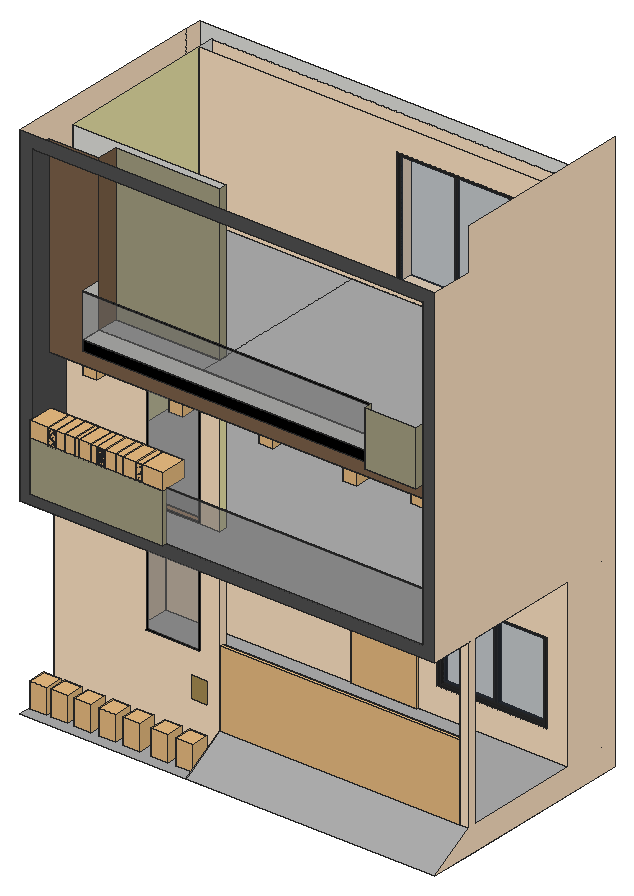
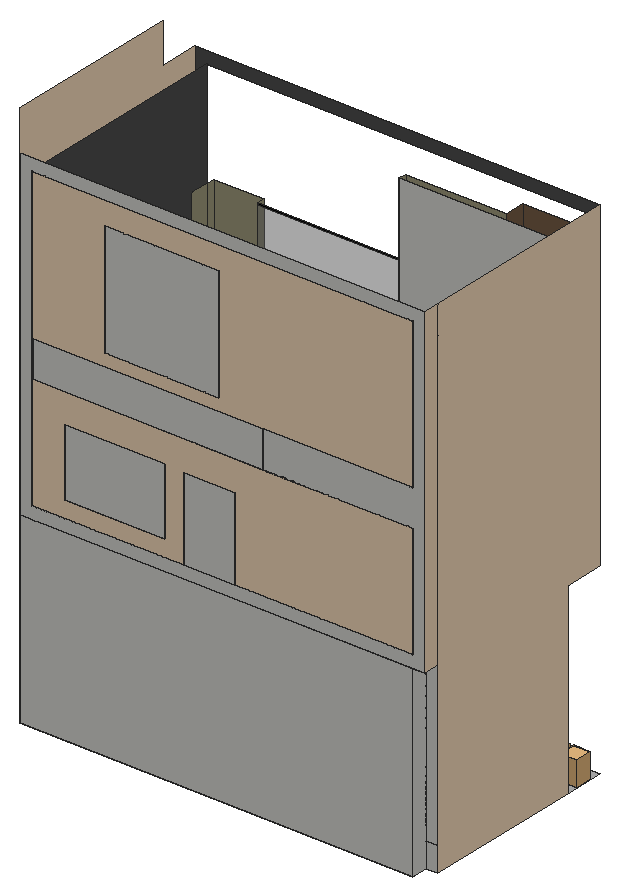
# SketchUp Ruby script. Lengths in inches.
U = 1.inch
M = Sketchup.active_model
def pt(a) = Geom::Point3d.new(a.map { |v| v * U })
def face(e, loops, mat)
  f = e.add_face(loops[0].map { |a| pt(a) })
  loops[1..].each { |l| e.add_face(l.map { |a| pt(a) }).erase! }
  f.material = f.back_material = mat if mat
  f
end
# faces: each face lists its corners as indices into pts; further lists are holes
def faces(e, pts, list, mat = nil) = list.each { |f| face(e, (f[0].is_a?(Array) ? f : [f]).map { |l| l.map { |i| pts[i] } }, mat) }
# xy, xz, yz: faces in a plane at the given z, y or x. An outline is a flat list of corners, or four numbers for a rectangle; further outlines are holes
def ring(l) = l.size == 4 ? [[l[0], l[1]], [l[2], l[1]], [l[2], l[3]], [l[0], l[3]]] : l.each_slice(2).to_a
def flat(e, list, mat, &to3) = list.each { |f| face(e, (f[0].is_a?(Array) ? f : [f]).map { |l| ring(l).map { |u, v| to3.(u, v) } }, mat) }
def xy(e, z, list, mat = nil) = flat(e, list, mat) { |x, y| [x, y, z] }
def xz(e, y, list, mat = nil) = flat(e, list, mat) { |x, z| [x, y, z] }
def yz(e, x, list, mat = nil) = flat(e, list, mat) { |y, z| [x, y, z] }
def lines(e, pts, list) = list.each { |a, b| e.add_line(pt(pts[a]), pt(pts[b])) }
# prism: a flat outline (further loops are holes) pulled along v
def prism(e, loops, v, mat = nil)
  f = face(e, loops, mat); d = Geom::Vector3d.new(v.map { |x| x * U })
  f.pushpull(f.normal.samedirection?(d) ? d.length : -d.length)
end
def box(e, o, s, mat = nil) = prism(e, [[o, [o[0] + s[0], o[1], o[2]], [o[0] + s[0], o[1] + s[1], o[2]], [o[0], o[1] + s[1], o[2]]]], [0, 0, s[2]], mat)
def at(x, y, z, deg = 0) = Geom::Transformation.translation(pt([x, y, z])) * Geom::Transformation.rotation(ORIGIN, Z_AXIS, deg.degrees)
def axes(o, x, y, z) = Geom::Transformation.new([*x, 0, *y, 0, *z, 0, *pt(o).to_a, 1])
def part(name) = M.definitions.add(name)
# library, detail: a bought-in or finely detailed component or shape, given as its bounding box
def library(name, o, s) = part(name).tap { |d| box(d.entities, o, s) }
def detail(e, o, s) = box(e.add_group.entities, o, s)
def put(e, d, t, mat = nil) = e.add_instance(d, t).tap { |i| i.material = mat if mat }
def group(e, t, mat = nil) = e.add_group.tap { |g| g.transformation = t; g.material = mat if mat }.entities
root = M.entities
M.materials.add("Translucent_Glass_Blue").color = [68, 104, 165]
M.materials["Translucent_Glass_Blue"].alpha = 0.07
M.materials.add("[0012_Bisque]").color = [255, 228, 196]
M.materials.add("[0048_PaleGoldenrod]").color = [238, 232, 170]
M.materials.add("[0054_LightYellow]").color = [255, 255, 224]
M.materials.add("[0061_OliveDrab]").color = [107, 142, 35]
M.materials.add("[0135_DarkGray]").color = [81, 81, 81]
M.materials.add("[0136_Charcoal]").color = [35, 35, 35]
M.materials.add("[0137_Black]").color = [0, 0, 0]
M.materials.add("[Brick Rough Tan]").color = [167, 141, 82]
M.materials.add("[Carrera Marble]").color = [175, 175, 175]
M.materials.add("[Cladding Siding Tan]").color = [124, 97, 73]
M.materials.add("[Cladding Siding Tan]1").color = [162, 126, 95]
M.materials.add("[Stone Coursed Rough]").color = [165, 160, 130]
M.materials.add("[Translucent Glass Gray]").color = [128, 128, 128]
M.materials["[Translucent Glass Gray]"].alpha = 0.5
M.materials.add("[Translucent_Glass_Green_Dark]").color = [33, 68, 103]
M.materials["[Translucent_Glass_Green_Dark]"].alpha = 0.08
c1 = library("Flower+pot",[-3.29,-4.11,0],[8.25,8.08,16.09])
c2 = library("Entrance door",[0,0,0],[5.9375,43.31,84.65])
c3 = library("Group\#4",[0,0,0],[120.6,5.32,84])
c4 = part("Glazed window sash")
xy(c4.entities,-18,[[0,-31,2,35]],"[0136_Charcoal]")
xy(c4.entities,-16,[[0,-29,0.9375,33],[0.9375,-29,1.125,33],[1.125,-29,2,1],[1.125,3,2,33]],"[0136_Charcoal]")
xy(c4.entities,76,[[0,-29,0.9375,33],[0.9375,-29,1.125,33],[1.125,-29,2,1],[1.125,3,2,33]],"[0136_Charcoal]")
xy(c4.entities,78,[[0,-31,2,35]],"[0136_Charcoal]")
xz(c4.entities,-31,[[0,-18,2,78]],"[0136_Charcoal]")
xz(c4.entities,-29,[[0,-16,0.9375,76],[0.9375,-16,1.125,76],[1.125,-16,2,76]],"[0136_Charcoal]")
xz(c4.entities,1,[[1.125,-16,2,76]],"[0136_Charcoal]")
xz(c4.entities,3,[[1.125,-16,2,76]],"[0136_Charcoal]")
xz(c4.entities,33,[[0,-16,0.9375,76],[0.9375,-16,1.125,76],[1.125,-16,2,76]],"[0136_Charcoal]")
xz(c4.entities,35,[[0,-18,2,78]],"[0136_Charcoal]")
yz(c4.entities,0,[[[-31,-18,35,78],[-29,-16,33,76]]],"[0136_Charcoal]")
yz(c4.entities,0.9375,[[-29,-16,33,76]],"Translucent_Glass_Blue")
yz(c4.entities,1.125,[[1,-16,3,76]],"[0136_Charcoal]")
yz(c4.entities,1.125,[[-29,-16,1,76],[3,-16,33,76]],"[Translucent_Glass_Green_Dark]")
yz(c4.entities,2,[[[-31,-18,35,78],[-29,-16,1,76],[3,-16,33,76]]],"[0136_Charcoal]")
c5 = part("Window assembly")
put(c5.entities,c4,axes([-31.84,50.72,0],[1,0,0],[0,1.1,0],[0,0,1]))
c6 = part("normal+window")
put(c6.entities,c5,axes([114.26,44.3125,18],[0,1,0],[-0.90909,0,0],[0,0,1]))
c7 = library("Ornamental grass",[0,0,0],[38.24,37.94,23.16])
c8 = library("Sphere Light\#4",[-9.875,-9.875,-9.875],[19.75,19.75,19.75])
c9 = library("Sphere Light\#5",[-10.1,-10.1,-10.1],[20.2,20.2,20.2])
c10 = library("Sphere Light\#6",[-10.32,-10.32,-10.32],[20.64,20.64,20.64])
c11 = library("Sphere Light\#3",[-9.875,-9.875,-9.875],[19.75,19.75,19.75])
c12 = library("Sphere Light\#7",[-9.875,-9.875,-9.875],[19.75,19.75,19.75])
xy(root,-36,[[240,12,600,72],[0,72,0,312,18,312,18,336,600,336,600,72]])
xy(root,-36,[[0,12,240,72]],"[Carrera Marble]")
xy(root,0,[[240,72,588,72,588,84,600,84,600,252,18,252,18,84,240,84]],"[Carrera Marble]")
xy(root,240,[[588,72,600,84],[0,312,18,336]])
xy(root,240,[[0,12,0,72,240,72,240,84,18,84,18,252,600,252,600,84,588,84,588,72,600,72,600,12]],"[Cladding Siding Tan]1")
xy(root,258,[[18,6,210.8,12],[281.21,312,356.77,336]])
xy(root,258,[[18,312,281.21,336],[356.77,312,582,336]],"[0012_Bisque]")
xy(root,258,[[18,12,582,12,582,312,18,312,18,84,240,84,240,72,18,72]],"[Carrera Marble]")
xy(root,283.21,[[385.84,312,533.22,336]],"[0012_Bisque]")
xy(root,330,[[18,6,210.8,12]],"[Stone Coursed Rough]")
xy(root,380.26,[[281.21,312,356.77,336]],"[0012_Bisque]")
xy(root,382.28,[[385.84,312,533.22,336]],"[0012_Bisque]")
xy(root,426.28,[[18,312,240,336],[240,312,580.875,336],[580.875,312,582,336]],"[0012_Bisque]")
xy(root,426.28,[[74.8,44.51,72.25,44.84,69.86,45.83,67.82,47.4,66.25,49.44,65.26,51.83,64.93,54.38,65.26,56.9375,66.25,59.32,67.82,61.36,69.86,62.93,72.25,63.92,74.8,64.26,77.36,63.92,79.74,62.93,81.78,61.36,83.35,59.32,84.34,56.9375,84.68,54.38,84.34,51.83,83.35,49.44,81.78,47.4,79.74,45.83,77.36,44.84],[199.49,44.51,196.93,44.84,194.55,45.83,192.51,47.4,190.9375,49.44,189.95,51.83,189.61,54.38,189.95,56.9375,190.9375,59.32,192.51,61.36,194.55,62.93,196.93,63.92,199.49,64.26,202.05,63.92,204.43,62.93,206.47,61.36,208.04,59.32,209.03,56.9375,209.36,54.38,209.03,51.83,208.04,49.44,206.47,47.4,204.43,45.83,202.05,44.84],[327.86,44.51,325.31,44.84,322.93,45.83,320.88,47.4,319.3125,49.44,318.33,51.83,317.99,54.38,318.33,56.9375,319.3125,59.32,320.88,61.36,322.93,62.93,325.31,63.92,327.86,64.26,330.42,63.92,332.8,62.93,334.85,61.36,336.42,59.32,337.4,56.9375,337.74,54.38,337.4,51.83,336.42,49.44,334.85,47.4,332.8,45.83,330.42,44.84],[450.49,44.51,447.93,44.84,445.55,45.83,443.51,47.4,441.9375,49.44,440.95,51.83,440.61,54.38,440.95,56.9375,441.9375,59.32,443.51,61.36,445.55,62.93,447.93,63.92,450.49,64.26,453.05,63.92,455.43,62.93,457.47,61.36,459.04,59.32,460.03,56.9375,460.36,54.38,460.03,51.83,459.04,49.44,457.47,47.4,455.43,45.83,453.05,44.84],[548.8,44.51,546.25,44.84,543.86,45.83,541.82,47.4,540.25,49.44,539.26,51.83,538.93,54.38,539.26,56.9375,540.25,59.32,541.82,61.36,543.86,62.93,546.25,63.92,548.8,64.26,551.36,63.92,553.74,62.93,555.78,61.36,557.35,59.32,558.34,56.9375,558.68,54.38,558.34,51.83,557.35,49.44,555.78,47.4,553.74,45.83,551.36,44.84]],"[0054_LightYellow]")
xy(root,426.28,[[[18,42,18,72,240,72,240,84,18,84,18,312,582,312,582,42],[199.49,44.51,202.05,44.84,204.43,45.83,206.47,47.4,208.04,49.44,209.03,51.83,209.36,54.38,209.03,56.9375,208.04,59.32,206.47,61.36,204.43,62.93,202.05,63.92,199.49,64.26,196.93,63.92,194.55,62.93,192.51,61.36,190.9375,59.32,189.95,56.9375,189.61,54.38,189.95,51.83,190.9375,49.44,192.51,47.4,194.55,45.83,196.93,44.84],[327.86,44.51,330.42,44.84,332.8,45.83,334.85,47.4,336.42,49.44,337.4,51.83,337.74,54.38,337.4,56.9375,336.42,59.32,334.85,61.36,332.8,62.93,330.42,63.92,327.86,64.26,325.31,63.92,322.93,62.93,320.88,61.36,319.3125,59.32,318.33,56.9375,317.99,54.38,318.33,51.83,319.3125,49.44,320.88,47.4,322.93,45.83,325.31,44.84],[450.49,44.51,453.05,44.84,455.43,45.83,457.47,47.4,459.04,49.44,460.03,51.83,460.36,54.38,460.03,56.9375,459.04,59.32,457.47,61.36,455.43,62.93,453.05,63.92,450.49,64.26,447.93,63.92,445.55,62.93,443.51,61.36,441.9375,59.32,440.95,56.9375,440.61,54.38,440.95,51.83,441.9375,49.44,443.51,47.4,445.55,45.83,447.93,44.84],[548.8,44.51,551.36,44.84,553.74,45.83,555.78,47.4,557.35,49.44,558.34,51.83,558.68,54.38,558.34,56.9375,557.35,59.32,555.78,61.36,553.74,62.93,551.36,63.92,548.8,64.26,546.25,63.92,543.86,62.93,541.82,61.36,540.25,59.32,539.26,56.9375,538.93,54.38,539.26,51.83,540.25,49.44,541.82,47.4,543.86,45.83,546.25,44.84],[74.8,44.51,77.36,44.84,79.74,45.83,81.78,47.4,83.35,49.44,84.34,51.83,84.68,54.38,84.34,56.9375,83.35,59.32,81.78,61.36,79.74,62.93,77.36,63.92,74.8,64.26,72.25,63.92,69.86,62.93,67.82,61.36,66.25,59.32,65.26,56.9375,64.93,54.38,65.26,51.83,66.25,49.44,67.82,47.4,69.86,45.83,72.25,44.84]]],"[0135_DarkGray]")
xy(root,465.19,[[507.27,12.12,507.27,42,90,42,89.95,12.79]])
xy(root,465.19,[[581.93,0,507.25,0.12,507.27,12.12,507.27,42,582,42,582,12.12,581.95,12.12]],"[Stone Coursed Rough]")
xy(root,480,[[507.27,12.12,507.27,42,90,42,89.95,12.79],[507.27,12.12,581.95,12.12,582,41.21,582,42,507.27,42],[581.95,12.12,582,12.12,582,41.21],[18,312,240,336],[240,312,580.875,336]])
xy(root,480,[[580.875,312,582,336]],"[0012_Bisque]")
xy(root,480,[[90,42,240,72],[240,42,582,312],[18,84,240,312]],"[Carrera Marble]")
xy(root,498,[[304.95,312,474.45,336]],"[0012_Bisque]")
xz(root,6,[[18,258,210.8,330]],"[Stone Coursed Rough]")
xz(root,12,[[18,258,210.8,330]])
xz(root,12,[[[0,240,600,720],[18,258,582,702]]],"[0135_DarkGray]")
xz(root,12,[[18,330,210.8,332],[210.8,330,582,332]],"[0137_Black]")
xz(root,12,[[210.8,258,582,330]],"[Translucent Glass Gray]")
xz(root,12.12,[[581.95,465.19,582,480]])
xz(root,42,[[90,465.19,240,480],[240,465.19,507.27,480],[507.27,465.19,582,480]])
xz(root,42,[[18,426.28,582,426.28,582,465.19,90,465.19,90,702,18,702]],"[Cladding Siding Tan]")
xz(root,72,[[18,426.28,240,426.28,240,480,90,480]])
xz(root,72,[[[0,-36,240,-36,240,240,212.66,240,212.66,92.87,134.29,92.87,134.29,240,0,240],[198.43,25.97,222.75,58.54]],[588,0,600,240],[18,258,134.29,258,134.29,419.18,212.66,419.18,212.66,258,240,258,240,426.28,18,426.28]],"[0012_Bisque]")
xz(root,72,[[[134.29,92.87,212.66,240],[136.29,94.87,210.66,238]],[[134.29,258,212.66,419.18],[136.29,260,210.66,417.18]]],"[0137_Black]")
xz(root,72,[[198.43,25.97,222.75,58.54]],"[Brick Rough Tan]")
xz(root,72,[[90,480,240,702]],"[Stone Coursed Rough]")
xz(root,84,[[18,480,240,702]])
xz(root,84,[[588,0,600,240]],"[0048_PaleGoldenrod]")
xz(root,84,[[18,0,240,240],[18,258,240,426.28]],"[Translucent Glass Gray]")
xz(root,252,[[[18,0,286.5,0,286.5,155.33,382.5,155.33,382.5,0,600,0,600,240,18,240],[410.96,39.28,569.52,157.78]]],"[0012_Bisque]")
xz(root,312,[[0,-36,18,0],[0,0,18,240],[240,426.28,580.875,480],[580.875,426.28,582,480]])
xz(root,312,[[[18,258,281.21,258,281.21,380.26,356.77,380.26,356.77,258,582,258,582,426.28,18,426.28],[385.84,283.21,533.22,382.28]],[[18,480,582,702],[304.95,498,474.45,667.5]]],"[0012_Bisque]")
xz(root,336,[[18,-36,600,240],[[0,240,600,720],[18,258,582,258,582,702,18,702,18,480,240,480,240,426.28,18,426.28]],[281.21,258,356.77,380.26],[385.84,283.21,533.22,382.28],[240,426.28,580.875,480],
  [304.95,498,474.45,667.5]])
xz(root,336,[[[18,258,18,426.28,582,426.28,582,258,356.77,258,356.77,380.26,281.21,380.26,281.21,258],[385.84,283.21,533.22,382.28]],[[18,480,582,702],[304.95,498,474.45,667.5]]],"[0012_Bisque]")
yz(root,0,[[72,-36,72,240,12,240,12,720,312,720,312,-36],[312,240,336,720]],"[0012_Bisque]")
yz(root,18,[[312,-36,336,240],[252,0,312,240],[312,480,336,702]])
yz(root,18,[[84,0,252,240],[312,258,336,426.28]],"[0012_Bisque]")
yz(root,18,[[84,258,312,426.28],[84,480,312,702]],"[0048_PaleGoldenrod]")
yz(root,18,[[12,258,72,258,72,426.28,42,426.28,42,702,12,702]],"[0135_DarkGray]")
yz(root,18,[[6,258,12,330]],"[Stone Coursed Rough]")
yz(root,89.95,[[12.79,541.57,42,543.57]],"[0137_Black]")
yz(root,90,[[42,480,72,702]],"[Cladding Siding Tan]")
yz(root,210.8,[[6,258,12,330]],"[Stone Coursed Rough]")
yz(root,240,[[72,426.28,84,480],[312,426.28,336,480]])
yz(root,240,[[72,0,84,240]],"[0012_Bisque]")
yz(root,240,[[72,258,84,426.28]],"[0048_PaleGoldenrod]")
yz(root,240,[[12,-36,72,-36,72,0]],"[Carrera Marble]")
yz(root,240,[[72,480,84,702]],"[Stone Coursed Rough]")
yz(root,281.21,[[312,258,336,380.26]],"[0012_Bisque]")
yz(root,304.95,[[312,498,336,667.5]],"[0012_Bisque]")
yz(root,356.77,[[312,258,336,380.26]],"[0012_Bisque]")
yz(root,385.84,[[312,283.21,336,382.28]],"[0012_Bisque]")
yz(root,474.45,[[312,498,336,667.5]],"[0012_Bisque]")
yz(root,507.27,[[12.12,465.19,42,480]])
yz(root,533.22,[[312,283.21,336,382.28]],"[0012_Bisque]")
yz(root,580.875,[[312,426.28,336,480]])
yz(root,582,[[42,426.28,72,480],[72,426.28,312,480],[312,426.28,336,480],[12.12,465.19,42,480],[312,480,336,702]])
yz(root,582,[[312,258,336,426.28]],"[0012_Bisque]")
yz(root,582,[[12,258,12,480,12.12,480,12.12,465.19,42,465.19,42,426.28,312,426.28,312,258],[12,480,312,702]],"[0135_DarkGray]")
yz(root,588,[[72,0,84,240]],"[0012_Bisque]")
yz(root,600,[[12,-36,336,-36,336,780,72,780,72,720,12,720,12,240,252,240,252,0,84,0,84,240,72,240,72,0]],"[0012_Bisque]")
p = [[600,72,0],[588,72,0],[240,72,0],[240,12,-36],[600,12,-36],[581.93,0,543.57],
  [507.25,0.12,543.57],[507.25,0.12,465.19],[581.93,0,465.19],[582,41.21,480],[582,41.21,543.57],[581.95,12.12,543.57],
  [581.95,12,543.57],[581.95,12.12,465.19],[581.95,12.12,480],[507.27,12.12,480],[507.27,12.12,465.19],[507.27,12.12,543.57],
  [507.27,12.12,541.57],[89.95,12.79,480],[89.95,12.79,465.19],[90,42,480],[90,42,465.19],[89.95,12.79,541.57],
  [90,42,543.57],[89.95,12.79,543.57],[582,12.12,465.19],[89.95,42,480],[89.95,12.12,480],[18,312,0],
  [600,312,0],[600,312,240],[18,312,240],[18,84,0],[18,84,-36],[382.5,252,0],
  [382.5,252,-36],[286.5,252,0],[286.5,252,-36],[18,252,0],[18,252,-36],[588,84,0],
  [588,84,-36],[1039.76,176.79,0],[1039.76,176.79,4.0625]]
faces(root,p,[[0,1,2,3,4]],"[Carrera Marble]")
faces(root,p,[[5,6,7,8],[9,10,11,12,5,8,13,14],[15,16,7,6,17,18]],"[Stone Coursed Rough]")
faces(root,p,[[16,15,19,20],[20,19,21,22],[25,23,18,17]],"[0137_Black]")
faces(root,p,[[23,19,15,18]],"[Translucent Glass Gray]")
faces(root,p,[[24,21,19,23,25]])
lines(root,p,[[26,12],[27,19],[15,28],[29,30],[31,32],[33,34],[35,36],[37,38],[39,40],[41,42],[43,44]])
put(root,c1,axes([40.86,41.03,-36],[2.97562,0,0],[0,3.14,0],[0,0,2.24147]))
put(root,c1,axes([74.92,41.03,-36],[2.97562,0,0],[0,3.14,0],[0,0,2.24147]))
put(root,c1,axes([111.04,41.03,-36],[2.97562,0,0],[0,3.14,0],[0,0,2.24147]))
put(root,c1,axes([145.67,41.03,-36],[2.97562,0,0],[0,3.14,0],[0,0,2.24147]))
put(root,c1,axes([186.23,41.03,-36],[2.97562,0,0],[0,3.14,0],[0,0,2.24147]))
put(root,c1,axes([221.67,41.03,-36],[2.97562,0,0],[0,3.14,0],[0,0,2.24147]))
put(root,c1,axes([11.04,41.03,-36],[2.97562,0,0],[0,3.14,0],[0,0,2.24147]))
put(root,c2,axes([286.5,256.9375,0],[0,-1,0],[2.21673,0,0],[0,0,1.83508]))
put(root,c3,axes([240,72,0],[2.88557,0,0],[0,1,0],[0,0,1.31]))
put(root,c6,axes([331.32,177.18,39.28],[2.40246,0,0],[0,6,0],[0,0,1.23438]))
put(root,c2,axes([281.21,317.9375,258],[0,-1,0],[1.74481,0,0],[0,0,1.44441]))
put(root,c6,axes([311.82,237.18,283.21],[2.23295,0,0],[0,6,0],[0,0,1.0319]))
put(root,c7,at(18,6,330),"[0061_OliveDrab]")
put(root,c7,at(45.25,6,330),"[0061_OliveDrab]")
put(root,c7,at(68.625,6,330),"[0061_OliveDrab]")
put(root,c7,at(89.3125,6,330),"[0061_OliveDrab]")
put(root,c7,at(115,6,330),"[0061_OliveDrab]")
put(root,c7,at(142.6875,6,330),"[0061_OliveDrab]")
put(root,c7,at(172.5625,6,330),"[0061_OliveDrab]")
put(root,c8,at(450.49,54.38,416.4))
put(root,c9,at(198.58,54.55,417.53))
put(root,c10,at(327.26,56.9375,421.12))
put(root,c11,at(74.8,54.38,421.34))
put(root,c12,at(548.8,54.74,421.34))
put(root,c6,axes([219.8125,299.53,498],[2.56818,0,0],[0,1,0],[0,0,1.76563]))
